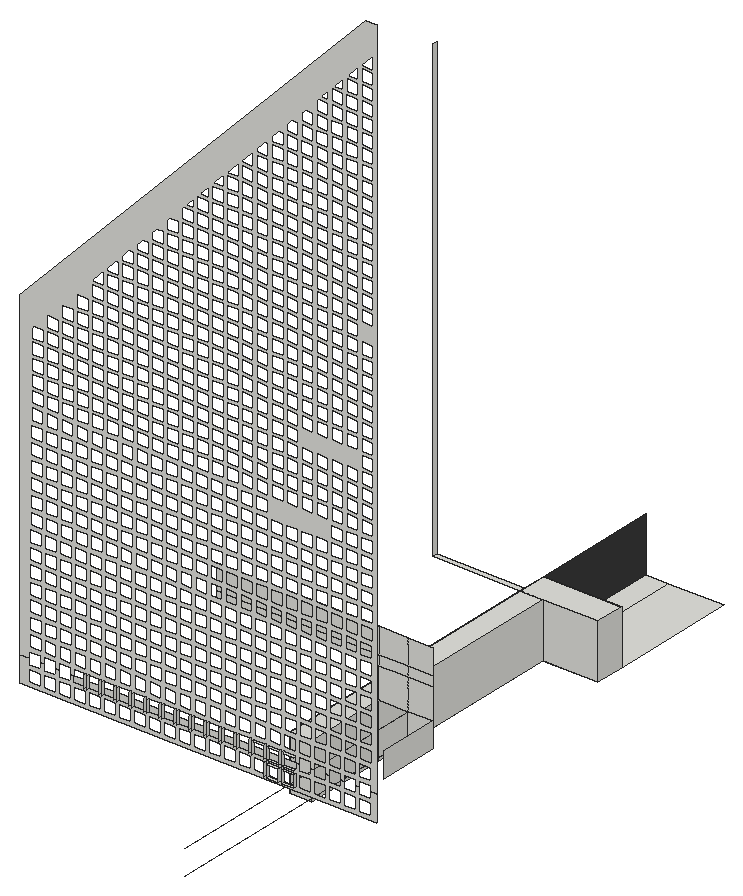
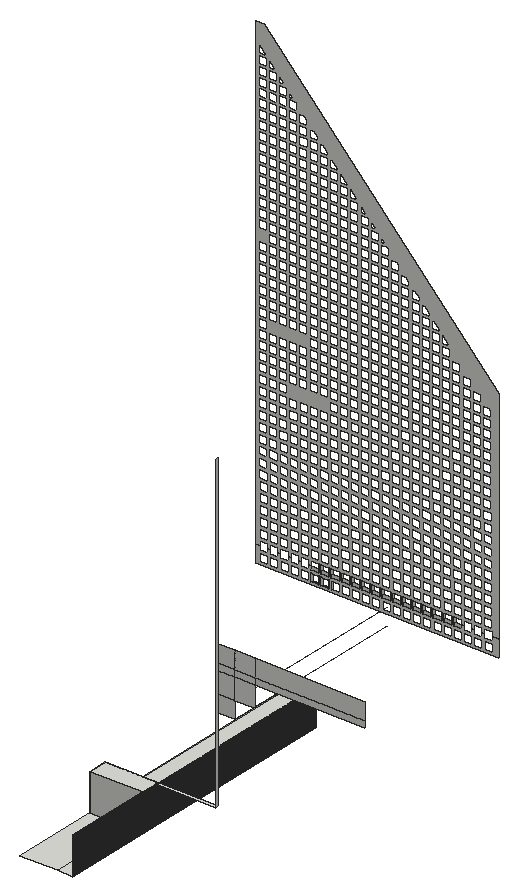
# SketchUp Ruby script. Lengths in inches.
U = 1.inch
M = Sketchup.active_model
def pt(a) = Geom::Point3d.new(a.map { |v| v * U })
def face(e, loops, mat)
  f = e.add_face(loops[0].map { |a| pt(a) })
  loops[1..].each { |l| e.add_face(l.map { |a| pt(a) }).erase! }
  f.material = f.back_material = mat if mat
  f
end
# faces: each face lists its corners as indices into pts; further lists are holes
def faces(e, pts, list, mat = nil) = list.each { |f| face(e, (f[0].is_a?(Array) ? f : [f]).map { |l| l.map { |i| pts[i] } }, mat) }
# xy, xz, yz: faces in a plane at the given z, y or x. An outline is a flat list of corners, or four numbers for a rectangle; further outlines are holes
def ring(l) = l.size == 4 ? [[l[0], l[1]], [l[2], l[1]], [l[2], l[3]], [l[0], l[3]]] : l.each_slice(2).to_a
def flat(e, list, mat, &to3) = list.each { |f| face(e, (f[0].is_a?(Array) ? f : [f]).map { |l| ring(l).map { |u, v| to3.(u, v) } }, mat) }
def xy(e, z, list, mat = nil) = flat(e, list, mat) { |x, y| [x, y, z] }
def xz(e, y, list, mat = nil) = flat(e, list, mat) { |x, z| [x, y, z] }
def yz(e, x, list, mat = nil) = flat(e, list, mat) { |y, z| [x, y, z] }
def lines(e, pts, list) = list.each { |a, b| e.add_line(pt(pts[a]), pt(pts[b])) }
# prism: a flat outline (further loops are holes) pulled along v
def prism(e, loops, v, mat = nil)
  f = face(e, loops, mat); d = Geom::Vector3d.new(v.map { |x| x * U })
  f.pushpull(f.normal.samedirection?(d) ? d.length : -d.length)
end
def box(e, o, s, mat = nil) = prism(e, [[o, [o[0] + s[0], o[1], o[2]], [o[0] + s[0], o[1] + s[1], o[2]], [o[0], o[1] + s[1], o[2]]]], [0, 0, s[2]], mat)
def at(x, y, z, deg = 0) = Geom::Transformation.translation(pt([x, y, z])) * Geom::Transformation.rotation(ORIGIN, Z_AXIS, deg.degrees)
def axes(o, x, y, z) = Geom::Transformation.new([*x, 0, *y, 0, *z, 0, *pt(o).to_a, 1])
def part(name) = M.definitions.add(name)
# library, detail: a bought-in or finely detailed component or shape, given as its bounding box
def library(name, o, s) = part(name).tap { |d| box(d.entities, o, s) }
def detail(e, o, s) = box(e.add_group.entities, o, s)
def put(e, d, t, mat = nil) = e.add_instance(d, t).tap { |i| i.material = mat if mat }
def group(e, t, mat = nil) = e.add_group.tap { |g| g.transformation = t; g.material = mat if mat }.entities
root = M.entities
M.materials.add("[Color M07]").color = [58, 58, 58]
xy(root,240.47,[[1350.1,505.3125,1354.48,561.375],[1350.1,561.375,1354.48,567.01],[1354.48,561.375,1365.24,567.01],[1350.1,567.01,1354.48,591.8125],[1354.48,567.01,1365.24,591.8125]])
xy(root,251.0625,[[1350.1,505.3125,1354.48,561.375],[1333.06,561.375,1350.1,562.32],[1350.1,561.375,1365.24,567.01]])
xy(root,259.68,[[1365.79,480.14,1368.1,480.77],[1368.7,480.14,1371.02,480.77]])
xy(root,262,[[1365.79,480.14,1368.1,480.77],[1368.7,480.14,1371.02,480.77]])
xy(root,262.73,[[1365.82,480.14,1368.13,480.77],[1368.73,480.14,1371.04,480.77]])
xy(root,265.04,[[1362.91,480.14,1365.22,480.77],[1365.82,480.14,1368.13,480.77],[1368.73,480.14,1371.04,480.77]])
xz(root,480.77,[[[1317.4375,258.95,1317.4375,263.89,1319.23,263.89,1319.23,262.73,1321.54,262.73,1321.54,263.89,1322.14,263.89,1322.14,262.73,1324.45,262.73,1324.45,263.89,1325.05,263.89,1325.05,262.73,1327.36,262.73,1327.36,263.89,1327.96,263.89,1327.96,262.73,1330.28,262.73,1330.28,263.89,1330.875,263.89,1330.875,262.73,1333.1875,262.73,1333.1875,263.89,1333.79,263.89,1333.79,262.73,1336.1,262.73,1336.1,263.89,1336.7,263.89,1336.7,262.73,1339.01,262.73,1339.01,263.89,1339.61,263.89,1339.61,262.73,1341.92,262.73,1341.92,263.89,1342.52,263.89,1342.52,262.73,1344.84,262.73,1344.84,263.89,1345.44,263.89,1345.44,262.73,1347.75,262.73,1347.75,263.89,1348.35,263.89,1348.35,262.73,1350.66,262.73,1350.66,263.89,1351.26,263.89,1351.26,262.73,1353.57,262.73,1353.57,263.89,1354.17,263.89,1354.17,262.73,1356.48,262.73,1356.48,263.89,1357.08,263.89,1357.08,262.73,1359.4,262.73,1359.4,263.89,1360,263.89,1360,262.73,1362.31,262.73,1362.31,263.89,1362.91,263.89,1362.91,262.73,1365.22,262.73,1365.22,263.89,1365.82,263.89,1365.82,262.73,1368.13,262.73,1368.13,263.89,1368.73,263.89,1368.73,262.73,1371.04,262.73,1371.04,263.89,1371.64,263.89,1371.64,262.73,1373.96,262.73,1373.96,263.89,1374.56,263.89,1374.56,262.73,1376.87,262.73,1376.87,263.89,1377.47,263.89,1377.47,262.73,1379.78,262.73,1379.78,263.89,1380.38,263.89,1380.38,262.73,1382.69,262.73,1382.69,263.89,1383.29,263.89,1383.29,262.73,1385.6,262.73,1385.6,263.89,1386.75,263.89,1386.75,258.95],[1383.26,259.68,1385.58,262],[1380.35,259.68,1382.66,262],[1377.4375,259.68,1379.75,262],[1374.53,259.68,1376.84,262],[1371.61,259.68,1373.93,262],[1368.7,259.68,1371.02,262],[1365.79,259.68,1368.1,262],[1362.88,259.68,1365.19,262],[1359.97,259.68,1362.28,262],[1357.05,259.68,1359.37,262],[1354.14,259.68,1356.45,262],[1351.23,259.68,1353.54,262],[1348.32,259.68,1350.63,262],[1345.41,259.68,1347.72,262],[1342.49,259.68,1344.81,262],[1339.58,259.68,1341.89,262],[1336.67,259.68,1338.98,262],[1333.76,259.68,1336.07,262],[1330.85,259.68,1333.16,262],[1327.93,259.68,1330.25,262],[1325.02,259.68,1327.33,262],[1322.11,259.68,1324.42,262],[1319.2,259.68,1321.51,262]],[1327.96,262.73,1330.28,263.89],[1330.875,262.73,1333.1875,263.89],[1333.79,262.73,1336.1,263.89],[1336.7,262.73,1339.01,263.89],
  [1339.61,262.73,1341.92,263.89],[1342.52,262.73,1344.84,263.89],[1345.44,262.73,1347.75,263.89],[1348.35,262.73,1350.66,263.89],[1351.26,262.73,1353.57,263.89],
  [1354.17,262.73,1356.48,263.89],[1357.08,262.73,1359.4,263.89],[1360,262.73,1362.31,263.89],[1362.91,262.73,1365.22,263.89],[1365.82,262.73,1368.13,263.89],
  [1368.73,262.73,1371.04,263.89],[[1317.4375,263.89,1317.4375,326.5,1384.5,397.75,1386.75,397.75,1386.75,263.89,1385.6,263.89,1385.6,265.04,1383.29,265.04,1383.29,263.89,1382.69,263.89,1382.69,265.04,1380.38,265.04,1380.38,263.89,1379.78,263.89,1379.78,265.04,1377.47,265.04,1377.47,263.89,1376.87,263.89,1376.87,265.04,1374.56,265.04,1374.56,263.89,1373.96,263.89,1373.96,265.04,1371.64,265.04,1371.64,263.89,1371.04,263.89,1371.04,265.04,1368.73,265.04,1368.73,263.89,1368.13,263.89,1368.13,265.04,1365.82,265.04,1365.82,263.89,1365.22,263.89,1365.22,265.04,1362.91,265.04,1362.91,263.89,1362.31,263.89,1362.31,265.04,1360,265.04,1360,263.89,1359.4,263.89,1359.4,265.04,1357.08,265.04,1357.08,263.89,1356.48,263.89,1356.48,265.04,1354.17,265.04,1354.17,263.89,1353.57,263.89,1353.57,265.04,1351.26,265.04,1351.26,263.89,1350.66,263.89,1350.66,265.04,1348.35,265.04,1348.35,263.89,1347.75,263.89,1347.75,265.04,1345.44,265.04,1345.44,263.89,1344.84,263.89,1344.84,265.04,1342.52,265.04,1342.52,263.89,1341.92,263.89,1341.92,265.04,1339.61,265.04,1339.61,263.89,1339.01,263.89,1339.01,265.04,1336.7,265.04,1336.7,263.89,1336.1,263.89,1336.1,265.04,1333.79,265.04,1333.79,263.89,1333.1875,263.89,1333.1875,265.04,1330.875,265.04,1330.875,263.89,1330.28,263.89,1330.28,265.04,1327.96,265.04,1327.96,263.89,1327.36,263.89,1327.36,265.04,1325.05,265.04,1325.05,263.89,1324.45,263.89,1324.45,265.04,1322.14,265.04,1322.14,263.89,1321.54,263.89,1321.54,265.04,1319.23,265.04,1319.23,263.89],[1372.05,370.27,1374.39,372.59],[1383.73,386.84,1386.04,389.15],[1383.73,384.09,1386.04,386.4],[1380.81,384.09,1383.13,386.4],[1380.79,381.34,1383.1,383.65],[1383.73,381.34,1386.04,383.65],[1383.73,378.59,1386.04,380.9],[1380.79,378.59,1383.1,380.9],[1377.88,375.84,1380.19,378.15],[1380.81,375.84,1383.13,378.15],[1383.73,375.84,1386.04,378.15],[1383.73,373.09,1386.04,375.4],[1380.79,373.09,1383.1,375.4],[1377.9,373.09,1380.22,375.4],[1374.97,373.09,1377.28,375.4],[1380.79,370.27,1383.1,372.59],[1383.73,370.27,1386.04,372.59],[1374.99,370.27,1377.3,372.59],[1369.17,370.27,1371.48,372.59],[1366.25,367.46,1368.57,369.77],[1369.17,367.46,1371.48,369.77],[1372.08,367.46,1374.39,369.77],[1374.99,367.46,1377.3,369.77],[1377.9,367.46,1380.22,369.77],[1380.81,367.46,1383.13,369.77],[1383.73,367.46,1386.04,369.77],[1383.73,364.65,1386.04,366.96],[1380.81,364.65,1383.13,366.96],[1377.9,364.65,1380.22,366.96],[1374.99,364.65,1377.3,366.96],[1372.08,364.65,1374.39,366.96],[1369.17,364.65,1371.48,366.96],[1366.25,364.65,1368.57,366.96],[1363.34,364.65,1365.65,366.96],[1360.43,361.84,1362.74,364.15],[1363.34,361.84,1365.65,364.15],[1366.25,361.84,1368.57,364.15],[1369.17,361.84,1371.48,364.15],[1372.08,361.84,1374.39,364.15],[1374.99,361.84,1377.3,364.15],[1377.9,361.84,1380.22,364.15],[1380.81,361.84,1383.13,364.15],[1383.73,361.84,1386.04,364.15],[1383.73,359.02,1386.04,361.34],[1380.81,359.02,1383.13,361.34],[1377.9,359.02,1380.22,361.34],[1374.99,359.02,1377.3,361.34],[1372.08,359.02,1374.39,361.34],[1369.17,359.02,1371.48,361.34],[1366.25,359.02,1368.57,361.34],[1363.34,359.02,1365.65,361.34],[1360.43,359.02,1362.74,361.34],[1357.52,359.02,1359.83,361.34],[1354.61,356.21,1356.92,358.52],[1357.52,356.21,1359.83,358.52],[1360.43,356.21,1362.74,358.52],[1363.34,356.21,1365.65,358.52],[1366.25,356.21,1368.57,358.52],[1369.17,356.21,1371.48,358.52],[1372.08,356.21,1374.39,358.52],[1374.99,356.21,1377.3,358.52],[1377.9,356.21,1380.22,358.52],[1380.81,356.21,1383.13,358.52],[1383.73,356.21,1386.04,358.52],[1351.69,350.59,1354.01,352.9],[1354.61,353.4,1356.92,355.71],[1354.61,350.59,1356.92,352.9],[1357.52,350.59,1359.83,352.9],[1357.52,353.4,1359.83,355.71],[1360.43,353.4,1362.74,355.71],[1360.43,350.59,1362.74,352.9],[1363.34,353.4,1365.65,355.71],[1363.34,350.59,1365.65,352.9],[1366.25,353.4,1368.57,355.71],[1366.25,350.59,1368.57,352.9],[1369.17,353.4,1371.48,355.71],[1369.17,350.59,1371.48,352.9],[1372.08,353.4,1374.39,355.71],[1372.08,350.59,1374.39,352.9],[1374.99,350.59,1377.3,352.9],[1374.99,353.4,1377.3,355.71],[1377.9,353.4,1380.22,355.71],[1380.81,353.4,1383.13,355.71],[1383.73,353.4,1386.04,355.71],[1383.73,350.59,1386.04,352.9],[1380.81,350.59,1383.13,352.9],[1377.9,350.59,1380.22,352.9],[1383.73,347.77,1386.04,350.09],[1380.81,347.77,1383.13,350.09],[1377.9,347.77,1380.22,350.09],[1374.99,347.77,1377.3,350.09],[1372.08,347.77,1374.39,350.09],[1369.17,347.77,1371.48,350.09],[1366.25,347.77,1368.57,350.09],[1363.34,347.77,1365.65,350.09],[1360.43,347.77,1362.74,350.09],[1357.52,347.77,1359.83,350.09],[1354.61,347.77,1356.92,350.09],[1351.69,347.77,1354.01,350.09],[1348.78,347.77,1351.09,350.09],[1345.87,344.96,1348.18,347.27],[1348.78,344.96,1351.09,347.27],[1351.69,344.96,1354.01,347.27],[1354.61,344.96,1356.92,347.27],[1357.52,344.96,1359.83,347.27],[1360.43,344.96,1362.74,347.27],[1363.34,344.96,1365.65,347.27],[1366.25,344.96,1368.57,347.27],[1369.17,344.96,1371.48,347.27],[1372.08,344.96,1374.39,347.27],[1374.99,344.96,1377.3,347.27],[1377.9,344.96,1380.22,347.27],[1380.81,344.96,1383.13,347.27],[1383.73,344.96,1386.04,347.27],[1337.13,336.52,1339.45,338.84],[1340.05,336.52,1342.36,338.84],[1342.96,336.52,1345.27,338.84],[1345.87,336.52,1348.18,338.84],[1348.78,336.52,1351.09,338.84],[1351.69,336.52,1354.01,338.84],[1354.61,336.52,1356.92,338.84],[1357.52,336.52,1359.83,338.84],[1360.43,336.52,1362.74,338.84],[1363.34,336.52,1365.65,338.84],[1363.34,339.34,1365.65,341.65],[1360.43,339.34,1362.74,341.65],[1357.52,339.34,1359.83,341.65],[1354.61,339.34,1356.92,341.65],[1351.69,339.34,1354.01,341.65],[1348.78,339.34,1351.09,341.65],[1345.87,339.34,1348.18,341.65],[1342.96,339.34,1345.27,341.65],[1340.05,339.34,1342.36,341.65],[1342.96,342.15,1345.27,344.46],[1345.87,342.15,1348.18,344.46],[1348.78,342.15,1351.09,344.46],[1351.69,342.15,1354.01,344.46],[1354.61,342.15,1356.92,344.46],[1357.52,342.15,1359.83,344.46],[1360.43,342.15,1362.74,344.46],[1363.34,342.15,1365.65,344.46],[1366.25,342.15,1368.57,344.46],[1366.25,339.34,1368.57,341.65],[1366.25,336.52,1368.57,338.84],[1369.17,336.52,1371.48,338.84],[1369.17,339.34,1371.48,341.65],[1369.17,342.15,1371.48,344.46],[1372.08,342.15,1374.39,344.46],[1372.08,339.34,1374.39,341.65],[1372.08,336.52,1374.39,338.84],[1374.99,336.52,1377.3,338.84],[1374.99,339.34,1377.3,341.65],[1374.99,342.15,1377.3,344.46],[1377.9,342.15,1380.22,344.46],[1377.9,339.34,1380.22,341.65],[1377.9,336.52,1380.22,338.84],[1380.81,336.52,1383.13,338.84],[1380.81,339.34,1383.13,341.65],[1380.81,342.15,1383.13,344.46],[1383.73,339.34,1386.04,341.65],[1383.73,336.52,1386.04,338.84],[1383.73,333.71,1386.04,336.02],[1380.81,333.71,1383.13,336.02],[1377.9,333.71,1380.22,336.02],[1374.99,333.71,1377.3,336.02],[1372.08,333.71,1374.39,336.02],[1369.17,333.71,1371.48,336.02],[1366.25,333.71,1368.57,336.02],[1363.34,333.71,1365.65,336.02],[1360.43,333.71,1362.74,336.02],[1357.52,333.71,1359.83,336.02],[1354.61,333.71,1356.92,336.02],[1351.69,333.71,1354.01,336.02],[1348.78,333.71,1351.09,336.02],[1345.87,333.71,1348.18,336.02],[1342.96,333.71,1345.27,336.02],[1340.05,333.71,1342.36,336.02],[1337.13,333.71,1339.45,336.02],[1334.22,333.71,1336.53,336.02],[1331.31,330.9,1333.62,333.21],[1334.22,330.9,1336.53,333.21],[1337.13,330.9,1339.45,333.21],[1340.05,330.9,1342.36,333.21],[1342.96,330.9,1345.27,333.21],[1345.87,330.9,1348.18,333.21],[1348.78,330.9,1351.09,333.21],[1351.69,330.9,1354.01,333.21],[1354.61,330.9,1356.92,333.21],[1357.52,330.9,1359.83,333.21],[1360.43,330.9,1362.74,333.21],[1363.34,330.9,1365.65,333.21],[1366.25,330.9,1368.57,333.21],[1369.17,330.9,1371.48,333.21],[1372.08,330.9,1374.39,333.21],[1374.99,330.9,1377.3,333.21],[1377.9,330.9,1380.22,333.21],[1380.81,330.9,1383.13,333.21],[1383.73,330.9,1386.04,333.21],[1383.73,328.09,1386.04,330.4],[1380.81,328.09,1383.13,330.4],[1377.9,328.09,1380.22,330.4],[1374.99,328.09,1377.3,330.4],[1372.08,328.09,1374.39,330.4],[1369.17,328.09,1371.48,330.4],[1366.25,328.09,1368.57,330.4],[1363.34,328.09,1365.65,330.4],[1360.43,328.09,1362.74,330.4],[1357.52,328.09,1359.83,330.4],[1354.61,328.09,1356.92,330.4],[1351.69,328.09,1354.01,330.4],[1348.78,328.09,1351.09,330.4],[1345.87,328.09,1348.18,330.4],[1342.96,328.09,1345.27,330.4],[1340.05,328.09,1342.36,330.4],[1337.13,328.09,1339.45,330.4],[1334.22,328.09,1336.53,330.4],[1331.31,328.09,1333.62,330.4],[1328.4,328.09,1330.71,330.4],[1325.49,325.27,1327.8,327.59],[1328.4,325.27,1330.71,327.59],[1331.31,325.27,1333.62,327.59],[1334.22,325.27,1336.53,327.59],[1337.13,325.27,1339.45,327.59],[1340.05,325.27,1342.36,327.59],[1342.96,325.27,1345.27,327.59],[1345.87,325.27,1348.18,327.59],[1348.78,325.27,1351.09,327.59],[1351.69,325.27,1354.01,327.59],[1354.61,325.27,1356.92,327.59],[1357.52,325.27,1359.83,327.59],[1360.43,325.27,1362.74,327.59],[1363.34,325.27,1365.65,327.59],[1366.25,325.27,1368.57,327.59],[1369.17,325.27,1371.48,327.59],[1372.08,325.27,1374.39,327.59],[1374.99,325.27,1377.3,327.59],[1377.9,325.27,1380.22,327.59],[1380.81,325.27,1383.13,327.59],[1383.73,325.27,1386.04,327.59],[1383.73,322.46,1386.04,324.77],[1380.81,322.46,1383.13,324.77],[1377.9,322.46,1380.22,324.77],[1374.99,322.46,1377.3,324.77],[1372.08,322.46,1374.39,324.77],[1369.17,322.46,1371.48,324.77],[1366.25,322.46,1368.57,324.77],[1363.34,322.46,1365.65,324.77],[1360.43,322.46,1362.74,324.77],[1357.52,322.46,1359.83,324.77],[1354.61,322.46,1356.92,324.77],[1351.69,322.46,1354.01,324.77],[1348.78,322.46,1351.09,324.77],[1345.87,322.46,1348.18,324.77],[1345.87,319.65,1348.18,321.96],[1348.78,319.65,1351.09,321.96],[1351.69,319.65,1354.01,321.96],[1354.61,319.65,1356.92,321.96],[1357.52,319.65,1359.83,321.96],[1360.43,319.65,1362.74,321.96],[1363.34,319.65,1365.65,321.96],[1366.25,319.65,1368.57,321.96],[1369.17,319.65,1371.48,321.96],[1383.73,319.65,1386.04,321.96],[1383.73,316.84,1386.04,319.15],[1380.81,316.84,1383.13,319.15],[1377.9,316.84,1380.22,319.15],[1374.99,316.84,1377.3,319.15],[1372.08,316.84,1374.39,319.15],[1369.17,316.84,1371.48,319.15],[1366.25,316.84,1368.57,319.15],[1363.34,316.84,1365.65,319.15],[1360.43,316.84,1362.74,319.15],[1357.52,316.84,1359.83,319.15],[1354.61,316.84,1356.92,319.15],[1351.69,316.84,1354.01,319.15],[1348.78,316.84,1351.09,319.15],[1345.87,316.84,1348.18,319.15],[1345.87,314.02,1348.18,316.34],[1348.78,314.02,1351.09,316.34],[1351.69,314.02,1354.01,316.34],[1354.61,314.02,1356.92,316.34],[1357.52,314.02,1359.83,316.34],[1360.43,314.02,1362.74,316.34],[1363.34,314.02,1365.65,316.34],[1366.25,314.02,1368.57,316.34],[1369.17,314.02,1371.48,316.34],[1372.08,314.02,1374.39,316.34],[1374.99,314.02,1377.3,316.34],[1377.9,314.02,1380.22,316.34],[1380.81,314.02,1383.13,316.34],[1383.73,314.02,1386.04,316.34],[1325.49,322.46,1327.8,324.77],[1328.4,322.46,1330.71,324.77],[1331.31,322.46,1333.62,324.77],[1334.22,322.46,1336.53,324.77],[1337.13,322.46,1339.45,324.77],[1340.05,322.46,1342.36,324.77],[1342.96,322.46,1345.27,324.77],[1342.96,319.65,1345.27,321.96],[1342.96,316.84,1345.27,319.15],[1342.96,314.02,1345.27,316.34],[1340.05,314.02,1342.36,316.34],[1340.05,316.84,1342.36,319.15],[1340.05,319.65,1342.36,321.96],[1337.13,319.65,1339.45,321.96],[1334.22,319.65,1336.53,321.96],[1331.31,319.65,1333.62,321.96],[1328.4,319.65,1330.71,321.96],[1325.49,319.65,1327.8,321.96],[1322.57,319.65,1324.89,321.96],[1319.66,316.84,1321.97,319.15],[1322.57,316.84,1324.89,319.15],[1325.49,316.84,1327.8,319.15],[1328.4,316.84,1330.71,319.15],[1331.31,316.84,1333.62,319.15],[1334.22,316.84,1336.53,319.15],[1337.13,316.84,1339.45,319.15],[1337.13,314.02,1339.45,316.34],[1334.22,314.02,1336.53,316.34],[1331.31,314.02,1333.62,316.34],[1328.4,314.02,1330.71,316.34],[1325.49,314.02,1327.8,316.34],[1322.57,314.02,1324.89,316.34],[1319.66,314.02,1321.97,316.34],[1319.66,311.21,1321.97,313.52],[1322.57,311.21,1324.89,313.52],[1325.49,311.21,1327.8,313.52],[1328.4,311.21,1330.71,313.52],[1331.31,311.21,1333.62,313.52],[1334.22,311.21,1336.53,313.52],[1337.13,311.21,1339.45,313.52],[1340.05,311.21,1342.36,313.52],[1342.96,311.21,1345.27,313.52],[1345.87,311.21,1348.18,313.52],[1348.78,311.21,1351.09,313.52],[1351.69,311.21,1354.01,313.52],[1354.61,311.21,1356.92,313.52],[1357.52,311.21,1359.83,313.52],[1360.43,311.21,1362.74,313.52],[1363.34,311.21,1365.65,313.52],[1366.25,311.21,1368.57,313.52],[1369.17,311.21,1371.48,313.52],[1372.08,311.21,1374.39,313.52],[1374.99,311.21,1377.3,313.52],[1377.9,311.21,1380.22,313.52],[1380.81,311.21,1383.13,313.52],[1383.73,311.21,1386.04,313.52],[1319.66,308.4,1321.97,310.71],[1322.57,308.4,1324.89,310.71],[1325.49,308.4,1327.8,310.71],[1328.4,308.4,1330.71,310.71],[1331.31,308.4,1333.62,310.71],[1334.22,308.4,1336.53,310.71],[1337.13,308.4,1339.45,310.71],[1340.05,308.4,1342.36,310.71],[1342.96,308.4,1345.27,310.71],[1345.87,308.4,1348.18,310.71],[1348.78,308.4,1351.09,310.71],[1351.69,308.4,1354.01,310.71],[1354.61,308.4,1356.92,310.71],[1357.52,308.4,1359.83,310.71],[1360.43,308.4,1362.74,310.71],[1363.34,308.4,1365.65,310.71],[1366.25,308.4,1368.57,310.71],[1369.17,308.4,1371.48,310.71],[1372.08,308.4,1374.39,310.71],[1374.99,308.4,1377.3,310.71],[1377.9,308.4,1380.22,310.71],[1380.81,308.4,1383.13,310.71],[1383.73,308.4,1386.04,310.71],[1383.7,305.35,1386.01,307.67],[1380.79,305.35,1383.1,307.67],[1377.875,305.35,1380.1875,307.67],[1363.3125,305.35,1365.625,307.67],[1360.4,305.35,1362.71,307.67],[1357.49,305.35,1359.8,307.67],[1354.58,305.35,1356.89,307.67],[1351.67,305.35,1353.98,307.67],[1348.75,305.35,1351.07,307.67],[1345.84,305.35,1348.15,307.67],[1342.93,305.35,1345.24,307.67],[1340.02,305.35,1342.33,307.67],[1337.11,305.35,1339.42,307.67],[1334.19,305.35,1336.51,307.67],[1331.28,305.35,1333.59,307.67],[1328.37,305.35,1330.68,307.67],[1325.46,305.35,1327.77,307.67],[1322.54,305.35,1324.86,307.67],[1319.63,305.35,1321.95,307.67],[1319.6,302.31,1321.92,304.62],[1322.52,302.31,1324.83,304.62],[1325.43,302.31,1327.74,304.62],[1328.34,302.31,1330.65,304.62],[1331.25,302.31,1333.56,304.62],[1334.16,302.31,1336.48,304.62],[1337.08,302.31,1339.39,304.62],[1339.99,302.31,1342.3,304.62],[1342.9,302.31,1345.21,304.62],[1345.8125,302.31,1348.125,304.62],[1348.72,302.31,1351.04,304.62],[1351.64,302.31,1353.95,304.62],[1354.55,302.31,1356.86,304.62],[1357.46,302.31,1359.77,304.62],[1360.37,302.31,1362.68,304.62],[1363.28,302.31,1365.6,304.62],[1366.2,302.31,1368.51,304.62],[1369.11,302.31,1371.42,304.62],[1372.02,302.31,1374.33,304.62],[1374.93,302.31,1377.25,304.62],[1377.84,302.31,1380.16,304.62],[1380.76,302.31,1383.07,304.62],[1383.67,302.31,1385.98,304.62],[1383.64,299.27,1385.95,301.58],[1380.73,299.27,1383.04,301.58],[1377.82,299.27,1380.13,301.58],[1374.9,299.27,1377.22,301.58],[1371.99,299.27,1374.3,301.58],[1369.08,299.27,1371.39,301.58],[1366.17,299.27,1368.48,301.58],[1363.26,299.27,1365.57,301.58],[1360.34,299.27,1362.66,301.58],[1357.43,299.27,1359.74,301.58],[1354.52,299.27,1356.83,301.58],[1351.61,299.27,1353.92,301.58],[1348.7,299.27,1351.01,301.58],[1345.78,299.27,1348.1,301.58],[1342.87,299.27,1345.18,301.58],[1339.96,299.27,1342.27,301.58],[1337.05,299.27,1339.36,301.58],[1334.14,299.27,1336.45,301.58],[1331.22,299.27,1333.54,301.58],[1328.3125,299.27,1330.625,301.58],[1325.4,299.27,1327.71,301.58],[1322.49,299.27,1324.8,301.58],[1319.57,299.27,1321.89,301.58],[1319.55,296.22,1321.86,298.53],[1322.46,296.22,1324.77,298.53],[1325.37,296.22,1327.68,298.53],[1328.28,296.22,1330.59,298.53],[1331.19,296.22,1333.51,298.53],[1334.11,296.22,1336.42,298.53],[1337.02,296.22,1339.33,298.53],[1339.93,296.22,1342.24,298.53],[1342.84,296.22,1345.15,298.53],[1345.75,296.22,1348.07,298.53],[1348.67,296.22,1350.98,298.53],[1351.58,296.22,1353.89,298.53],[1354.49,296.22,1356.8,298.53],[1357.4,296.22,1359.71,298.53],[1360.3125,296.22,1362.625,298.53],[1363.23,296.22,1365.54,298.53],[1366.14,296.22,1368.45,298.53],[1369.05,296.22,1371.36,298.53],[1371.96,296.22,1374.28,298.53],[1374.875,296.22,1377.1875,298.53],[1377.79,296.22,1380.1,298.53],[1380.7,296.22,1383.01,298.53],[1383.61,296.22,1385.92,298.53],[1319.52,293.18,1321.83,295.49],[1322.43,293.18,1324.74,295.49],[1325.34,293.18,1327.65,295.49],[1328.25,293.18,1330.57,295.49],[1331.17,293.18,1333.48,295.49],[1334.08,293.18,1336.39,295.49],[1336.99,293.18,1339.3,295.49],[1339.9,293.18,1342.21,295.49],[1342.8125,293.18,1345.125,295.49],[1345.73,293.18,1348.04,295.49],[1348.64,293.18,1350.95,295.49],[1351.55,293.18,1353.86,295.49],[1354.46,293.18,1356.77,295.49],[1357.375,293.18,1359.6875,295.49],[1360.29,293.18,1362.6,295.49],[1363.2,293.18,1365.51,295.49],[1366.11,293.18,1368.42,295.49],[1369.02,293.18,1371.33,295.49],[1371.93,293.18,1374.25,295.49],[1374.85,293.18,1377.16,295.49],[1377.76,293.18,1380.07,295.49],[1380.67,293.18,1382.98,295.49],[1383.58,293.18,1385.89,295.49],[1331.14,290.13,1333.45,292.44],[1334.05,290.13,1336.36,292.44],[1336.96,290.13,1339.27,292.44],[1339.87,290.13,1342.18,292.44],[1342.78,290.13,1345.1,292.44],[1345.7,290.13,1348.01,292.44],[1348.61,290.13,1350.92,292.44],[1351.52,290.13,1353.83,292.44],[1354.43,290.13,1356.74,292.44],[1357.34,290.13,1359.66,292.44],[1360.26,290.13,1362.57,292.44],[1363.17,290.13,1365.48,292.44],[1366.08,290.13,1368.39,292.44],[1368.99,290.13,1371.31,292.44],[1371.9,290.13,1374.22,292.44],[1374.82,290.13,1377.13,292.44],[1377.73,290.13,1380.04,292.44],[1380.64,290.13,1382.95,292.44],[1383.55,290.13,1385.87,292.44],[1383.52,287.09,1385.84,289.4],[1380.61,287.09,1382.92,289.4],[1377.7,287.09,1380.01,289.4],[1374.79,287.09,1377.1,289.4],[1371.875,287.09,1374.1875,289.4],[1368.96,287.09,1371.28,289.4],[1366.05,287.09,1368.36,289.4],[1363.14,287.09,1365.45,289.4],[1360.23,287.09,1362.54,289.4],[1357.32,287.09,1359.63,289.4],[1354.4,287.09,1356.72,289.4],[1351.49,287.09,1353.8,289.4],[1348.58,287.09,1350.89,289.4],[1345.67,287.09,1347.98,289.4],[1342.76,287.09,1345.07,289.4],[1339.84,287.09,1342.16,289.4],[1336.93,287.09,1339.24,289.4],[1334.02,287.09,1336.33,289.4],[1331.11,287.09,1333.42,289.4],[1331.08,284.04,1333.39,286.35],[1333.99,284.04,1336.3,286.35],[1336.9,284.04,1339.21,286.35],[1339.8125,284.04,1342.125,286.35],[1342.73,284.04,1345.04,286.35],[1345.64,284.04,1347.95,286.35],[1348.55,284.04,1350.86,286.35],[1351.46,284.04,1353.77,286.35],[1354.375,284.04,1356.6875,286.35],[1357.29,284.04,1359.6,286.35],[1360.2,284.04,1362.51,286.35],[1363.11,284.04,1365.42,286.35],[1366.02,284.04,1368.34,286.35],[1368.93,284.04,1371.25,286.35],[1371.85,284.04,1374.16,286.35],[1374.76,284.04,1377.07,286.35],[1377.67,284.04,1379.98,286.35],[1380.58,284.04,1382.9,286.35],[1383.49,284.04,1385.81,286.35],[1383.47,281,1385.78,283.31],[1380.55,281,1382.87,283.31],[1377.64,281,1379.95,283.31],[1374.73,281,1377.04,283.31],[1371.82,281,1374.13,283.31],[1368.91,281,1371.22,283.31],[1365.99,281,1368.31,283.31],[1363.08,281,1365.39,283.31],[1360.17,281,1362.48,283.31],[1357.26,281,1359.57,283.31],[1354.35,281,1356.66,283.31],[1351.43,281,1353.75,283.31],[1348.52,281,1350.83,283.31],[1345.61,281,1347.92,283.31],[1342.7,281,1345.01,283.31],[1339.79,281,1342.1,283.31],[1336.875,281,1339.1875,283.31],[1333.96,281,1336.27,283.31],[1333.93,277.95,1336.24,280.26],[1336.84,277.95,1339.16,280.26],[1339.76,277.95,1342.07,280.26],[1342.67,277.95,1344.98,280.26],[1345.58,277.95,1347.89,280.26],[1348.49,277.95,1350.8,280.26],[1351.4,277.95,1353.72,280.26],[1354.32,277.95,1356.63,280.26],[1357.23,277.95,1359.54,280.26],[1360.14,277.95,1362.45,280.26],[1363.05,277.95,1365.36,280.26],[1365.96,277.95,1368.28,280.26],[1368.875,277.95,1371.1875,280.26],[1371.79,277.95,1374.1,280.26],[1374.7,277.95,1377.01,280.26],[1377.61,277.95,1379.93,280.26],[1380.52,277.95,1382.84,280.26],[1383.4375,277.95,1385.75,280.26],[1383.41,274.91,1385.72,277.22],[1380.5,274.91,1382.81,277.22],[1377.58,274.91,1379.9,277.22],[1374.67,274.91,1376.98,277.22],[1371.76,274.91,1374.07,277.22],[1368.85,274.91,1371.16,277.22],[1365.9375,274.91,1368.25,277.22],[1363.02,274.91,1365.34,277.22],[1360.11,274.91,1362.42,277.22],[1357.2,274.91,1359.51,277.22],[1354.29,274.91,1356.6,277.22],[1351.375,274.91,1353.6875,277.22],[1348.46,274.91,1350.78,277.22],[1345.55,274.91,1347.86,277.22],[1342.64,274.91,1344.95,277.22],[1339.73,274.91,1342.04,277.22],[1336.82,274.91,1339.13,277.22],[1333.9,274.91,1336.22,277.22],[1331.05,281,1333.36,283.31],[1331.02,277.95,1333.33,280.26],[1330.99,274.91,1333.3,277.22],[1328.08,274.91,1330.39,277.22],[1328.11,277.95,1330.42,280.26],[1328.14,281,1330.45,283.31],[1328.17,284.04,1330.48,286.35],[1328.2,287.09,1330.51,289.4],[1328.22,290.13,1330.54,292.44],[1325.3125,290.13,1327.625,292.44],[1325.28,287.09,1327.6,289.4],[1325.25,284.04,1327.57,286.35],[1325.23,281,1327.54,283.31],[1322.28,277.95,1324.6,280.26],[1325.2,277.95,1327.51,280.26],[1325.17,274.91,1327.48,277.22],[1322.25,274.91,1324.57,277.22],[1322.3125,281,1324.625,283.31],[1322.34,284.04,1324.65,286.35],[1322.37,287.09,1324.68,289.4],[1322.4,290.13,1324.71,292.44],[1319.49,290.13,1321.8,292.44],[1319.46,287.09,1321.77,289.4],[1319.43,284.04,1321.74,286.35],[1319.4,281,1321.71,283.31],[1319.37,277.95,1321.68,280.26],[1319.34,274.91,1321.66,277.22],[1319.3125,271.86,1321.625,274.17],[1322.23,271.86,1324.54,274.17],[1325.14,271.86,1327.45,274.17],[1328.05,271.86,1330.36,274.17],[1330.96,271.86,1333.27,274.17],[1333.875,271.86,1336.1875,274.17],[1336.79,271.86,1339.1,274.17],[1339.7,271.86,1342.01,274.17],[1342.61,271.86,1344.92,274.17],[1345.52,271.86,1347.83,274.17],[1348.43,271.86,1350.75,274.17],[1351.35,271.86,1353.66,274.17],[1354.26,271.86,1356.57,274.17],[1357.17,271.86,1359.48,274.17],[1360.08,271.86,1362.39,274.17],[1362.99,271.86,1365.31,274.17],[1365.91,271.86,1368.22,274.17],[1368.82,271.86,1371.13,274.17],[1371.73,271.86,1374.04,274.17],[1374.64,271.86,1376.96,274.17],[1377.55,271.86,1379.87,274.17],[1380.47,271.86,1382.78,274.17],[1383.38,271.86,1385.69,274.17],[1383.35,268.82,1385.66,271.13],[1380.4375,268.82,1382.75,271.13],[1377.53,268.82,1379.84,271.13],[1374.61,268.82,1376.93,271.13],[1371.7,268.82,1374.01,271.13],[1368.79,268.82,1371.1,271.13],[1365.88,268.82,1368.19,271.13],[1362.97,268.82,1365.28,271.13],[1360.05,268.82,1362.37,271.13],[1357.14,268.82,1359.45,271.13],[1354.23,268.82,1356.54,271.13],[1351.32,268.82,1353.63,271.13],[1348.41,268.82,1350.72,271.13],[1345.49,268.82,1347.81,271.13],[1342.58,268.82,1344.89,271.13],[1339.67,268.82,1341.98,271.13],[1336.76,268.82,1339.07,271.13],[1333.85,268.82,1336.16,271.13],[1330.93,268.82,1333.25,271.13],[1328.02,268.82,1330.33,271.13],[1325.11,268.82,1327.42,271.13],[1322.2,268.82,1324.51,271.13],[1319.28,268.82,1321.6,271.13],[1319.26,265.77,1321.57,268.09],[1322.17,265.77,1324.48,268.09],[1325.08,265.77,1327.39,268.09],[1327.99,265.77,1330.3,268.09],[1330.9,265.77,1333.22,268.09],[1333.82,265.77,1336.13,268.09],[1336.73,265.77,1339.04,268.09],[1339.64,265.77,1341.95,268.09],[1342.55,265.77,1344.86,268.09],[1345.46,265.77,1347.78,268.09],[1348.375,265.77,1350.6875,268.09],[1351.29,265.77,1353.6,268.09],[1354.2,265.77,1356.51,268.09],[1357.11,265.77,1359.42,268.09],[1360.02,265.77,1362.34,268.09],[1362.9375,265.77,1365.25,268.09],[1365.85,265.77,1368.16,268.09],[1368.76,265.77,1371.07,268.09],[1371.67,265.77,1373.99,268.09],[1374.58,265.77,1376.9,268.09],[1377.5,265.77,1379.81,268.09],[1380.41,265.77,1382.72,268.09],[1383.32,265.77,1385.63,268.09],[1377.9,381.34,1380.22,381.34,1380.22,383.65,1378.01,383.65,1377.9,383.53],[1377.9,378.59,1380.22,378.59,1380.22,380.9,1378.01,380.9,1377.9,380.78],[1374.99,375.84,1377.3,375.84,1377.3,378.15,1375.1,378.15,1374.99,378.03],[1372.08,373.09,1374.39,373.09,1374.39,375.4,1372.1875,375.4,1372.08,375.28],[1377.9,370.27,1380.22,370.27,1380.22,372.59,1378.01,372.59,1377.9,372.47],[1351.69,353.4,1354.01,353.4,1354.01,355.71,1351.83,355.71,1351.69,355.57],[1322.57,322.46,1324.89,322.46,1324.89,324.77,1322.83,324.77,1322.57,324.5],[1348.78,350.59,1351.09,350.59,1351.09,352.9,1349.19,352.9,1348.78,352.46],[1374.99,378.59,1377.3,378.59,1377.3,380.9,1375.43,380.9,1374.99,380.43],[1319.66,319.65,1321.97,319.65,1321.97,321.96,1320.19,321.96,1319.66,321.39],[1345.87,347.77,1348.18,347.77,1348.18,350.09,1346.55,350.09,1345.87,349.36],[1372.08,375.84,1374.39,375.84,1374.39,378.15,1372.86,378.15,1372.08,377.32],[1342.96,344.96,1345.27,344.96,1345.27,347.27,1343.92,347.27,1342.96,346.25],[1369.17,373.09,1371.48,373.09,1371.48,375.4,1370.28,375.4,1369.17,374.21],[1340.05,342.15,1342.36,342.15,1342.36,344.46,1341.28,344.46,1340.05,343.14],[1366.25,370.27,1368.57,370.27,1368.57,372.59,1367.64,372.59,1366.25,371.11],[1337.13,339.34,1339.45,339.34,1339.45,341.65,1338.65,341.65,1337.13,340.04],[1363.34,367.46,1365.65,367.46,1365.65,369.77,1365.01,369.77,1363.34,368],[1334.22,336.52,1336.53,336.52,1336.53,338.84,1336.01,338.84,1334.22,336.93],[1360.43,364.65,1362.74,364.65,1362.74,366.96,1362.37,366.96,1360.43,364.89],[1383.73,389.59,1386.04,389.59,1386.04,391.9,1385.74,391.9,1383.73,389.75],[1331.31,333.71,1333.62,333.71,1333.62,336.02,1333.375,336.02,1331.31,333.82],[1357.57,361.84,1359.83,361.84,1359.83,364.15,1359.73,364.15],[1381,386.84,1383.13,386.84,1383.13,389.11],[1354.93,359.02,1356.92,359.02,1356.92,361.14],[1378.42,384.09,1380.22,384.09,1380.22,386],[1352.3,356.21,1354.01,356.21,1354.01,358.04],[1375.84,381.34,1377.3,381.34,1377.3,382.89],[1349.66,353.4,1351.09,353.4,1351.09,354.93]]])
xz(root,505.3125,[[1350.1,240.47,1354.48,251.0625]])
xz(root,521.5625,[[1360.2,246.25,1365.01,251.0625],[1354.48,251.0625,1360.2,257.0625],[1360.2,251.0625,1365.01,257.0625],[1322.96,257.0625,1354.48,258.95],[1354.48,257.0625,1360.2,258.95],
  [1360.2,257.0625,1365.01,258.95],[1322.96,258.95,1354.48,263.89],[1354.48,258.95,1360.2,263.89],[1360.2,258.95,1365.01,263.89]])
xz(root,561.375,[[1350.1,240.47,1354.48,251.0625],[1354.48,240.47,1365.24,251.0625]])
xz(root,567.01,[[1350.1,240.47,1365.24,251.0625]])
yz(root,1330.28,[[480.14,262.73,480.77,265.04]])
yz(root,1330.875,[[480.14,262.73,480.77,265.04]])
yz(root,1333.06,[[561.375,251.0625,562.32,340.125]])
yz(root,1333.1875,[[480.14,262.73,480.77,265.04]])
yz(root,1333.79,[[480.14,262.73,480.77,265.04]])
yz(root,1336.1,[[480.14,262.73,480.77,265.04]])
yz(root,1336.7,[[480.14,262.73,480.77,265.04]])
yz(root,1339.01,[[480.14,262.73,480.77,265.04]])
yz(root,1339.61,[[480.14,262.73,480.77,265.04]])
yz(root,1341.92,[[480.14,262.73,480.77,265.04]])
yz(root,1342.52,[[480.14,262.73,480.77,265.04]])
yz(root,1344.84,[[480.14,262.73,480.77,265.04]])
yz(root,1345.44,[[480.14,262.73,480.77,265.04]])
yz(root,1347.75,[[480.14,262.73,480.77,265.04]])
yz(root,1348.35,[[480.14,262.73,480.77,265.04]])
yz(root,1350.1,[[505.3125,240.47,561.375,251.0625],[561.375,240.47,567.01,251.0625],[567.01,240.47,591.8125,251.0625]],"[Color M07]")
yz(root,1350.66,[[480.14,262.73,480.77,265.04]])
yz(root,1351.26,[[480.14,262.73,480.77,265.04]])
yz(root,1353.57,[[480.14,262.73,480.77,265.04]])
yz(root,1354.17,[[480.14,262.73,480.77,265.04]])
yz(root,1354.48,[[505.3125,240.47,521.5625,251.0625],[521.5625,240.47,561.375,251.0625]])
yz(root,1356.48,[[480.14,262.73,480.77,265.04]])
yz(root,1357.08,[[480.14,262.73,480.77,265.04]])
yz(root,1359.4,[[480.14,262.73,480.77,265.04]])
yz(root,1360,[[480.14,262.73,480.77,265.04]])
yz(root,1362.31,[[480.14,262.73,480.77,265.04]])
yz(root,1362.91,[[480.14,262.73,480.77,265.04]])
yz(root,1365.01,[[509.6875,246.25,521.5625,251.0625]])
yz(root,1365.19,[[480.14,259.68,480.77,262]])
yz(root,1365.22,[[480.14,262.73,480.77,265.04]])
yz(root,1365.24,[[561.375,240.47,567.01,251.0625]])
yz(root,1365.79,[[480.14,259.68,480.77,262]])
yz(root,1365.82,[[480.14,262.73,480.77,265.04]])
yz(root,1368.1,[[480.14,259.68,480.77,262]])
yz(root,1368.13,[[480.14,262.73,480.77,265.04]])
yz(root,1368.7,[[480.14,259.68,480.77,262]])
yz(root,1368.73,[[480.14,262.73,480.77,265.04]])
yz(root,1371.02,[[480.14,259.68,480.77,262]])
p = [[1360.2,521.5625,251.0625],[1360.2,467.1875,251.0625],[1360.2,521.5625,246.25],[1360.2,467.1875,246.25]]
lines(root,p,[[0,1],[2,3]])
